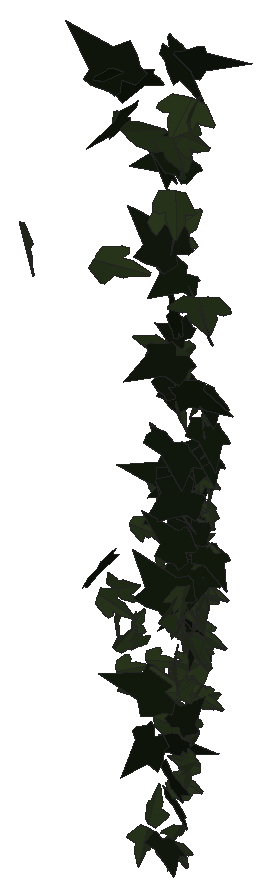
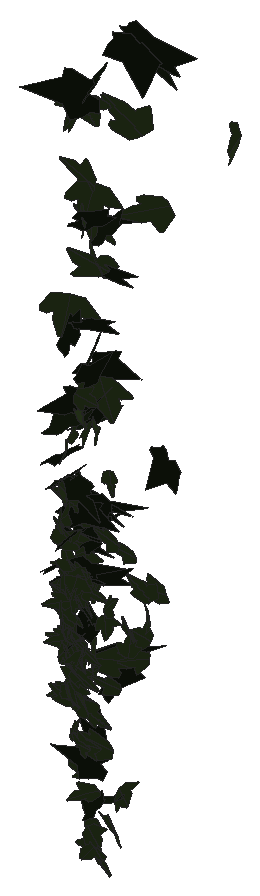
# SketchUp Ruby script. Lengths in inches.
U = 1.inch
M = Sketchup.active_model
def pt(a) = Geom::Point3d.new(a.map { |v| v * U })
def face(e, loops, mat)
  f = e.add_face(loops[0].map { |a| pt(a) })
  loops[1..].each { |l| e.add_face(l.map { |a| pt(a) }).erase! }
  f.material = f.back_material = mat if mat
  f
end
# faces: each face lists its corners as indices into pts; further lists are holes
def faces(e, pts, list, mat = nil) = list.each { |f| face(e, (f[0].is_a?(Array) ? f : [f]).map { |l| l.map { |i| pts[i] } }, mat) }
# xy, xz, yz: faces in a plane at the given z, y or x. An outline is a flat list of corners, or four numbers for a rectangle; further outlines are holes
def ring(l) = l.size == 4 ? [[l[0], l[1]], [l[2], l[1]], [l[2], l[3]], [l[0], l[3]]] : l.each_slice(2).to_a
def flat(e, list, mat, &to3) = list.each { |f| face(e, (f[0].is_a?(Array) ? f : [f]).map { |l| ring(l).map { |u, v| to3.(u, v) } }, mat) }
def xy(e, z, list, mat = nil) = flat(e, list, mat) { |x, y| [x, y, z] }
def xz(e, y, list, mat = nil) = flat(e, list, mat) { |x, z| [x, y, z] }
def yz(e, x, list, mat = nil) = flat(e, list, mat) { |y, z| [x, y, z] }
def lines(e, pts, list) = list.each { |a, b| e.add_line(pt(pts[a]), pt(pts[b])) }
# prism: a flat outline (further loops are holes) pulled along v
def prism(e, loops, v, mat = nil)
  f = face(e, loops, mat); d = Geom::Vector3d.new(v.map { |x| x * U })
  f.pushpull(f.normal.samedirection?(d) ? d.length : -d.length)
end
def box(e, o, s, mat = nil) = prism(e, [[o, [o[0] + s[0], o[1], o[2]], [o[0] + s[0], o[1] + s[1], o[2]], [o[0], o[1] + s[1], o[2]]]], [0, 0, s[2]], mat)
def at(x, y, z, deg = 0) = Geom::Transformation.translation(pt([x, y, z])) * Geom::Transformation.rotation(ORIGIN, Z_AXIS, deg.degrees)
def axes(o, x, y, z) = Geom::Transformation.new([*x, 0, *y, 0, *z, 0, *pt(o).to_a, 1])
def part(name) = M.definitions.add(name)
# library, detail: a bought-in or finely detailed component or shape, given as its bounding box
def library(name, o, s) = part(name).tap { |d| box(d.entities, o, s) }
def detail(e, o, s) = box(e.add_group.entities, o, s)
def put(e, d, t, mat = nil) = e.add_instance(d, t).tap { |i| i.material = mat if mat }
def group(e, t, mat = nil) = e.add_group.tap { |g| g.transformation = t; g.material = mat if mat }.entities
root = M.entities
M.materials.add("1026 AP 7946 SUNNY SIDE UP").color = [254, 231, 186]
M.materials.add("efeu1").color = [18, 25, 13]
M.materials.add("efeu2").color = [43, 57, 29]
c1 = part("ivyleaf_10")
p = [[0,0.5,-0.03],[-0.0625,2.02,-0.43],[-0.19,2.01,-0.46],[-0.54,1.05,-0.29],[-0.52,0.625,-0.18],[-0.83,0.76,-0.28],
  [-1.16,0.64,-0.33],[-1.15,0.33,-0.24],[-0.77,-0.39,0.02],[-0.3,-0.51,0.16],[0.04,-0.48,0.23],[-0.02,2.01,-0.4375],
  [-0.06,2.01,-0.43],[0.04,-0.49,0.23],[0.67,-0.49,0.14],[1.38,0.36,-0.2],[1.375,0.51,-0.24],[0.81,0.65,-0.19],
  [0.62,0.59,-0.15],[0.6,1.09,-0.28],[0.5,1.23,-0.31]]
faces(c1.entities,p,[[0,1,2,3,4,5,6,7,8,9,10],[11,12,0,13,14,15,16,17,18,19,20]],"efeu2")
c2 = part("ivyleaf_9")
p = [[1.54,2.16,1.25],[1.36,2.04,1.19],[-0.21,0.99,0.68],[-0.71,1.11,0.82],[-0.85,0.86,0.67],[-0.8,0.17,0.21],
  [-0.9,-0.01,0.1],[-0.67,-0.16,-0.02],[-0.08,-0.08,-0.05],[-0.03,-0.6,-0.4],[0.65,-0.88,-0.66],[0.83,-0.6,-0.49],
  [1.29,-0.42,-0.43],[1.8125,-0.07,-0.26],[1.21,0.44,0.15]]
faces(c2.entities,p,[[0,1,2,3,4,5,6,7,8,9,10,11,12,13,14]],"efeu1")
put(root,c1,axes([137.27,204.8,264.4375],[-0.21228,0.31455,-0.21083],[0.10791,-0.19506,-0.35356],[-0.58168,-0.15098,0.01135]),"1026 AP 7946 SUNNY SIDE UP")
put(root,c2,axes([138.43,205.78,256.27],[-0.14943,0.12354,-0.33542],[-0.27565,0.27548,0.16166],[0.47432,0.19902,-0.01172]),"1026 AP 7946 SUNNY SIDE UP")
put(root,c2,axes([138.74,206.35,267.0625],[-0.36936,0.26298,-0.15561],[0.1174,-0.13697,-0.3625],[-0.46341,-0.24431,0.0322]),"1026 AP 7946 SUNNY SIDE UP")
put(root,c1,axes([137.98,206.61,263.21],[-0.15297,-0.09398,-0.35608],[0.46781,0.17726,-0.13509],[0.31218,-0.31168,0.02796]),"1026 AP 7946 SUNNY SIDE UP")
put(root,c2,axes([138.58,207.46,251.5],[0.02682,-0.05486,-0.40252],[0.29455,-0.34272,0.05604],[-0.54547,-0.18777,0.01047]),"1026 AP 7946 SUNNY SIDE UP")
put(root,c2,axes([137.97,207.08,267.47],[-0.03931,0.10478,0.44908],[-0.49984,0.3029,-0.09214],[-0.49583,-0.31366,0.05728]),"1026 AP 7946 SUNNY SIDE UP")
put(root,c2,axes([138.1,207.17,267.54],[0.27569,0.29178,-0.14907],[-0.09098,-0.13573,-0.35095],[-0.50515,0.18368,-0.01815]),"1026 AP 7946 SUNNY SIDE UP")
put(root,c1,axes([138.1,207.79,248.85],[-0.05681,-0.25331,0.18976],[0.16619,-0.18576,-0.24103],[0.465,0.03545,0.10933]),"1026 AP 7946 SUNNY SIDE UP")
put(root,c1,axes([137.82,207.68,265.81],[-0.35908,-0.09139,0.2943],[0.45463,0.03082,0.24799],[-0.12835,0.36484,0.05505]),"1026 AP 7946 SUNNY SIDE UP")
put(root,c1,axes([137.11,207.7,254.25],[0.08937,0.02554,0.27361],[0.41558,0.03078,-0.06117],[-0.05589,0.26971,-0.01732]),"1026 AP 7946 SUNNY SIDE UP")
put(root,c2,axes([138.4,208,252.34],[-0.16035,-0.2823,-0.21493],[-0.10551,-0.19588,0.30806],[-0.54026,0.12204,0.00363]),"1026 AP 7946 SUNNY SIDE UP")
put(root,c1,axes([137.22,207.97,253.61],[-0.02174,0.04114,-0.24935],[0.1048,-0.23294,-0.04603],[-0.37193,-0.06804,0.0016]),"1026 AP 7946 SUNNY SIDE UP")
put(root,c1,axes([138.37,208.11,252.28],[-0.05152,0.0425,0.36196],[-0.31307,-0.29365,0.01575],[0.45962,-0.19525,0.0513]),"1026 AP 7946 SUNNY SIDE UP")
put(root,c2,axes([138.57,208.1875,258.29],[-0.07894,-0.35099,0.12447],[0.13846,-0.13162,-0.35122],[0.56808,-0.01669,0.1029]),"1026 AP 7946 SUNNY SIDE UP")
put(root,c2,axes([138.35,208.11,248.66],[-0.04833,-0.26842,0.06253],[0.14171,-0.06896,-0.261],[0.40942,-0.00781,0.09772]),"1026 AP 7946 SUNNY SIDE UP")
put(root,c1,axes([138.48,208.32,254.14],[0.01062,-0.05018,-0.36681],[-0.03601,-0.35517,0.04908],[-0.56381,0.02174,-0.01005]),"1026 AP 7946 SUNNY SIDE UP")
put(root,c2,axes([138.42,208.24,250.11],[0.07435,-0.07825,0.29064],[0.15266,-0.26589,-0.09415],[0.43502,0.10668,-0.01664]),"1026 AP 7946 SUNNY SIDE UP")
put(root,c1,axes([137.3125,207.95,253.1],[0.00959,-0.17395,0.17565],[-0.01251,0.17131,0.18031],[-0.38388,-0.00993,-0.00149]),"1026 AP 7946 SUNNY SIDE UP")
put(root,c1,axes([137.39,207.93,252.55],[0.02346,-0.01229,-0.25266],[0.24321,0.19122,0.00094],[0.29976,-0.15419,0.01902]),"1026 AP 7946 SUNNY SIDE UP")
put(root,c1,axes([137.14,208.11,254.33],[-0.25796,-0.01163,0.18737],[0.28374,0.02458,0.16938],[-0.04092,0.24375,-0.0067]),"1026 AP 7946 SUNNY SIDE UP")
put(root,c1,axes([138.48,208.48,248.2],[0.05216,-0.07558,0.20674],[0.08378,-0.19425,-0.08539],[0.32727,0.06177,-0.01109]),"1026 AP 7946 SUNNY SIDE UP")
put(root,c1,axes([138.76,208.4,266.45],[0.49856,0.13271,-0.10172],[-0.12513,-0.06662,-0.35318],[-0.22882,0.32557,-0.02851]),"1026 AP 7946 SUNNY SIDE UP")
put(root,c1,axes([137.41,208.43,252.96],[-0.12147,-0.17915,-0.06958],[-0.05431,-0.05748,0.20046],[-0.29553,0.08419,-0.00824]),"1026 AP 7946 SUNNY SIDE UP")
put(root,c1,axes([138.59,208.46,254.59],[-0.06434,-0.29395,0.07829],[0.11226,-0.08546,-0.29498],[0.4647,-0.02006,0.0821]),"1026 AP 7946 SUNNY SIDE UP")
put(root,c2,axes([138.61,208.45,255.63],[-0.2433,-0.28255,0.01311],[-0.00479,0.018,0.33177],[-0.44482,0.15435,-0.01075]),"1026 AP 7946 SUNNY SIDE UP")
put(root,c2,axes([138.47,208.375,254.44],[-0.47842,-0.18786,-0.0325],[-0.06268,0.00671,0.3674],[-0.29262,0.30571,-0.02557]),"1026 AP 7946 SUNNY SIDE UP")
put(root,c2,axes([138.2,208.64,260.1],[-0.00175,-0.01928,-0.36432],[-0.00079,-0.35353,0.0178],[-0.55672,0.00056,0.00112]),"1026 AP 7946 SUNNY SIDE UP")
put(root,c1,axes([137.35,208.43,253.39],[0.23057,-0.14791,-0.03381],[0.05167,-0.01234,0.21398],[-0.23227,-0.14957,0.01404]),"1026 AP 7946 SUNNY SIDE UP")
put(root,c2,axes([138.46,208.54,251.31],[-0.20919,0.18329,0.17464],[0.16876,-0.13014,0.2324],[0.35322,0.17073,-0.00761]),"1026 AP 7946 SUNNY SIDE UP")
put(root,c1,axes([138.45,208.38,252.74],[-0.08363,0.11263,0.31846],[-0.31206,0.23796,-0.12336],[-0.41143,-0.20338,0.02884]),"1026 AP 7946 SUNNY SIDE UP")
put(root,c1,axes([138.47,208.67,249.97],[-0.04252,-0.20025,0.02134],[0.07316,-0.02766,-0.20198],[0.30818,-0.02106,0.0509]),"1026 AP 7946 SUNNY SIDE UP")
put(root,c1,axes([137.17,208.6875,255.61],[0.00895,-0.03411,-0.21442],[0.30603,-0.07888,0.01836],[-0.12701,-0.19248,0.02912]),"1026 AP 7946 SUNNY SIDE UP")
put(root,c2,axes([138.48,208.8,256.82],[-0.58057,0.01593,-0.03948],[0.05748,-0.0392,-0.379],[-0.03116,-0.36914,0.03635]),"1026 AP 7946 SUNNY SIDE UP")
put(root,c1,axes([138.09,208.79,263.77],[0.52149,-0.09691,0.15922],[0.21566,-0.0807,-0.35453],[0.19025,0.35713,-0.03455]),"1026 AP 7946 SUNNY SIDE UP")
put(root,c1,axes([138.9,208.43,266.15],[-0.00558,0.03021,0.35349],[-0.21461,0.31475,-0.02818],[-0.49699,-0.13625,0.0082]),"1026 AP 7946 SUNNY SIDE UP")
put(root,c1,axes([138.43,208.61,249.625],[0.13704,0.21404,-0.06837],[0.02392,0.0667,0.23822],[0.35212,-0.08783,0.01043]),"1026 AP 7946 SUNNY SIDE UP")
put(root,c1,axes([138.38,208.68,253.75],[0.10194,-0.24117,-0.11016],[-0.03952,0.10254,-0.25666],[0.41206,0.0695,0.00263]),"1026 AP 7946 SUNNY SIDE UP")
put(root,c1,axes([138.36,208.78,252],[0.19521,-0.1543,-0.11315],[0.12625,-0.07491,0.2031],[-0.26885,-0.14721,0.01322]),"1026 AP 7946 SUNNY SIDE UP")
put(root,c1,axes([138.47,208.89,250.26],[-0.00801,0.05453,0.21713],[0.08596,-0.20343,0.05447],[0.33086,0.05417,-0.00889]),"1026 AP 7946 SUNNY SIDE UP")
put(root,c2,axes([138.16,208.6875,262.59],[-0.51837,-0.07034,-0.17757],[-0.27636,0.00448,0.34524],[-0.09474,0.3718,-0.0355]),"1026 AP 7946 SUNNY SIDE UP")
put(root,c2,axes([138.33,208.82,253.98],[-0.29779,0.13854,-0.10576],[0.11107,-0.07805,-0.24136],[-0.24815,-0.20119,0.01889]),"1026 AP 7946 SUNNY SIDE UP")
put(root,c1,axes([138.25,208.88,254.02],[0.09784,-0.00823,0.23936],[0.3392,-0.08777,-0.06322],[0.13651,0.22399,-0.01447]),"1026 AP 7946 SUNNY SIDE UP")
put(root,c2,axes([138.05,208.76,267.38],[0.36087,-0.28525,-0.21895],[-0.22656,0.1546,-0.37601],[0.50974,0.27066,-0.01211]),"1026 AP 7946 SUNNY SIDE UP")
put(root,c1,axes([138.47,208.84,251.4],[-0.35283,0.0622,0.10485],[0.16392,-0.00155,0.23858],[0.09016,0.24624,-0.02345]),"1026 AP 7946 SUNNY SIDE UP")
put(root,c1,axes([138.8,208.83,261.5],[-0.50005,-0.21165,-0.04949],[0.08921,-0.001,-0.39216],[0.32897,-0.32144,0.03111]),"1026 AP 7946 SUNNY SIDE UP")
put(root,c1,axes([137.88,209.04,263.09],[0.28789,-0.18585,0.2122],[0.21162,-0.15775,-0.26942],[0.38287,0.22694,-0.01064]),"1026 AP 7946 SUNNY SIDE UP")
put(root,c2,axes([137.87,209.04,249.07],[0.1098,-0.1935,0.14411],[0.06205,-0.13555,-0.21258],[0.3713,0.07987,-0.00709]),"1026 AP 7946 SUNNY SIDE UP")
put(root,c2,axes([137.99,208.9,259.16],[-0.1715,-0.24048,0.15713],[0.08622,0.14403,0.27274],[-0.44057,0.1218,-0.00779]),"1026 AP 7946 SUNNY SIDE UP")
put(root,c1,axes([138.01,209,248.43],[-0.08255,-0.19904,0.07055],[-0.01351,-0.06966,-0.21227],[0.33129,-0.05244,0.00892]),"1026 AP 7946 SUNNY SIDE UP")
put(root,c2,axes([138.11,208.96,256.86],[-0.20076,-0.07795,-0.23052],[-0.32185,-0.09077,0.15267],[-0.18639,0.2407,-0.01533]),"1026 AP 7946 SUNNY SIDE UP")
put(root,c1,axes([138.02,208.95,248.03],[-0.30631,0.03804,-0.0833],[0.11627,-0.04119,-0.20318],[-0.07945,-0.20694,0.02382]),"1026 AP 7946 SUNNY SIDE UP")
put(root,c1,axes([138.44,209.1,250.83],[-0.0274,0.05563,0.20616],[0.14152,-0.17861,0.05827],[0.29381,0.09122,-0.00884]),"1026 AP 7946 SUNNY SIDE UP")
put(root,c1,axes([138.47,208.98,253.125],[-0.38521,0.0857,-0.11891],[0.15772,-0.06281,-0.26661],[-0.1628,-0.26364,0.02307]),"1026 AP 7946 SUNNY SIDE UP")
put(root,c1,axes([138.47,209.02,253.18],[-0.29423,0.12034,-0.17806],[0.20782,-0.11408,-0.22899],[-0.25896,-0.22827,0.01854]),"1026 AP 7946 SUNNY SIDE UP")
put(root,c1,axes([138.08,209.05,256.44],[-0.03035,-0.0377,-0.25412],[0.34512,-0.11983,0.00048],[-0.18598,-0.21623,0.04236]),"1026 AP 7946 SUNNY SIDE UP")
put(root,c2,axes([138.17,208.84,259.2],[0.05089,0.00326,-0.32937],[0.24383,0.28089,0.02077],[0.43969,-0.15614,0.0266]),"1026 AP 7946 SUNNY SIDE UP")
put(root,c2,axes([138.48,208.85,255.64],[-0.52553,0.02145,-0.08664],[-0.12803,0.03973,0.34354],[0.04778,0.34237,-0.0324]),"1026 AP 7946 SUNNY SIDE UP")
put(root,c1,axes([137.92,208.92,247.87],[0.14845,-0.11689,-0.18783],[-0.20684,0.12614,-0.15331],[0.26943,0.16125,-0.01421]),"1026 AP 7946 SUNNY SIDE UP")
put(root,c1,axes([137.37,208.99,252.32],[0.09255,-0.02455,-0.20343],[0.31189,-0.00731,0.06185],[-0.02213,-0.20579,0.02085]),"1026 AP 7946 SUNNY SIDE UP")
put(root,c1,axes([137.41,208.93,248.5625],[0.3866,-0.19255,0.102],[-0.0914,0.08732,0.3206],[-0.32877,-0.25069,0.03081]),"1026 AP 7946 SUNNY SIDE UP")
put(root,c2,axes([138.38,209.29,260.89],[0.03261,-0.12433,0.39737],[0.08169,-0.38293,-0.13204],[0.63304,0.05582,-0.00343]),"1026 AP 7946 SUNNY SIDE UP")
put(root,c2,axes([138.14,209.12,253.43],[0.34432,-0.13217,0.017],[-0.00467,0.02834,0.26262],[-0.20953,-0.21782,0.02209]),"1026 AP 7946 SUNNY SIDE UP")
put(root,c1,axes([138.25,209.13,252.26],[-0.14705,-0.08734,-0.18617],[-0.21653,-0.11637,0.13104],[-0.22864,0.16638,-0.00436]),"1026 AP 7946 SUNNY SIDE UP")
put(root,c2,axes([137.9375,209.15,256.8],[-0.26336,0.02022,0.29029],[-0.4377,-0.06695,-0.16596],[0.07475,-0.32079,0.05097]),"1026 AP 7946 SUNNY SIDE UP")
put(root,c2,axes([138.39,209.18,254.79],[-0.27314,-0.2426,-0.05525],[0.07861,0.02826,-0.30624],[0.38221,-0.17918,0.0235]),"1026 AP 7946 SUNNY SIDE UP")
put(root,c1,axes([138.07,209,258.75],[-0.12102,0.27967,0.01811],[-0.02748,0.01176,-0.29842],[-0.43962,-0.07773,0.01367]),"1026 AP 7946 SUNNY SIDE UP")
put(root,c1,axes([138.39,209.07,250.09],[0.02983,-0.01261,-0.20835],[-0.31353,0.03459,-0.0213],[0.05608,0.20009,-0.00824]),"1026 AP 7946 SUNNY SIDE UP")
put(root,c1,axes([137.68,209.08,259.9],[-0.56075,-0.06376,0.13403],[-0.19072,-0.05944,-0.37182],[0.12556,-0.37506,0.03383]),"1026 AP 7946 SUNNY SIDE UP")
put(root,c1,axes([138.44,209.05,251.87],[-0.19637,-0.05084,-0.21241],[0.32776,0.01461,-0.13388],[0.06145,-0.24036,0.03531]),"1026 AP 7946 SUNNY SIDE UP")
put(root,c2,axes([138.03,209.2,255.81],[0.26522,-0.22788,0.09308],[-0.06293,0.08419,0.29203],[-0.38104,-0.17251,0.01655]),"1026 AP 7946 SUNNY SIDE UP")
put(root,c1,axes([137.33,209.26,254.44],[0.00113,0.02169,0.22004],[0.11205,-0.20137,0.01965],[0.31823,0.07083,-0.0077]),"1026 AP 7946 SUNNY SIDE UP")
put(root,c1,axes([138.37,209.2,253.33],[-0.00667,-0.19743,-0.10454],[-0.00697,-0.10028,0.20284],[-0.34817,0.00579,-0.00206]),"1026 AP 7946 SUNNY SIDE UP")
put(root,c1,axes([138.09,209.13,254.63],[-0.10759,0.00135,0.20859],[-0.30217,-0.06775,-0.06684],[0.10027,-0.2027,0.02241]),"1026 AP 7946 SUNNY SIDE UP")
put(root,c1,axes([137.53,209.16,250.82],[0.00838,-0.03053,-0.31371],[0.45089,-0.10543,0.01545],[-0.16737,-0.28555,0.02592]),"1026 AP 7946 SUNNY SIDE UP")
put(root,c2,axes([138,209.02,260.53],[-0.0697,-0.16956,0.25995],[0.07994,0.24826,0.18182],[-0.47256,0.067,-0.00758]),"1026 AP 7946 SUNNY SIDE UP")
put(root,c1,axes([137.76,208.97,262.82],[0.37546,0.07194,-0.27499],[0.35066,0.15922,0.25027],[0.25797,-0.32115,0.06004]),"1026 AP 7946 SUNNY SIDE UP")
put(root,c1,axes([138.38,209.17,252.47],[0.28959,-0.04065,-0.18182],[-0.28037,0.00158,-0.1923],[0.04792,0.25492,-0.02628]),"1026 AP 7946 SUNNY SIDE UP")
put(root,c1,axes([138.38,209.22,253.95],[0.28876,-0.09256,0.11789],[0.14727,-0.06875,-0.21156],[0.17936,0.20546,-0.0161]),"1026 AP 7946 SUNNY SIDE UP")
put(root,c1,axes([138.04,209.15,255.45],[-0.14781,-0.20461,-0.00666],[0.01645,0.00103,-0.23177],[0.32141,-0.09415,0.0088]),"1026 AP 7946 SUNNY SIDE UP")
put(root,c1,axes([138.53,209.18,252.02],[0.09617,-0.20196,0.00355],[-0.00711,-0.00617,-0.21734],[0.31757,0.06102,-0.00594]),"1026 AP 7946 SUNNY SIDE UP")
put(root,c1,axes([138.14,209.31,254.52],[-0.03365,-0.24586,0.17407],[0.14595,-0.16783,-0.23848],[0.44711,0.03628,0.09095]),"1026 AP 7946 SUNNY SIDE UP")
put(root,c1,axes([138.4375,209.15,251.99],[-0.31393,0.00268,0.13484],[-0.20426,-0.03339,-0.20366],[0.02529,-0.23637,0.02889]),"1026 AP 7946 SUNNY SIDE UP")
put(root,c1,axes([137.91,209.22,265.09],[-0.10024,0.05344,0.33373],[0.50792,-0.04715,0.07329],[0.08976,0.32648,-0.04204]),"1026 AP 7946 SUNNY SIDE UP")
put(root,c1,axes([138.51,209.13,251.66],[-0.20743,-0.06641,0.15099],[0.19357,0.08114,0.15211],[-0.16377,0.18003,-0.01145]),"1026 AP 7946 SUNNY SIDE UP")
put(root,c1,axes([137.4,209.11,257.72],[-0.23451,0.09458,0.10549],[-0.15171,0.03711,-0.18081],[-0.15733,-0.17675,0.01711]),"1026 AP 7946 SUNNY SIDE UP")
put(root,c1,axes([138.51,209.31,253.09],[-0.02854,-0.22591,0.12697],[0.12494,-0.12366,-0.2199],[0.38589,0.02333,0.08059]),"1026 AP 7946 SUNNY SIDE UP")
put(root,c1,axes([138.59,209.22,253.79],[0.05508,-0.26684,0.00737],[0.07168,-0.00264,-0.27339],[0.41363,0.03599,0.0464]),"1026 AP 7946 SUNNY SIDE UP")
put(root,c1,axes([137.63,209.33,258.85],[-0.06233,0.0565,-0.20028],[0.0231,-0.1971,-0.06314],[-0.31799,-0.02539,0.03467]),"1026 AP 7946 SUNNY SIDE UP")
put(root,c1,axes([138.32,209.23,253.28],[-0.12799,-0.00103,-0.25664],[0.37376,-0.07876,-0.08013],[-0.11723,-0.24996,0.0247]),"1026 AP 7946 SUNNY SIDE UP")
put(root,c2,axes([137.7,209.14,250.34],[0.25443,0.09029,-0.20688],[0.24878,0.12656,0.1902],[0.24184,-0.22517,0.022]),"1026 AP 7946 SUNNY SIDE UP")
put(root,c2,axes([138.16,209.28,255.18],[-0.14871,0.02877,0.25893],[-0.39737,-0.01848,-0.09595],[0.01145,-0.26775,0.03285]),"1026 AP 7946 SUNNY SIDE UP")
put(root,c2,axes([137.875,209.36,260.1],[0.01651,0.04137,0.27628],[-0.31028,-0.18272,0.03596],[0.29236,-0.19626,0.02257]),"1026 AP 7946 SUNNY SIDE UP")
put(root,c2,axes([138.22,208.97,267.11],[0.15505,0.19314,-0.30545],[0.14599,0.28406,0.22328],[0.53841,-0.13265,0.02742]),"1026 AP 7946 SUNNY SIDE UP")
put(root,c2,axes([138.24,209.3,253.04],[-0.2258,0.02543,-0.20214],[0.29315,-0.06431,-0.14942],[-0.10483,-0.23461,0.01755]),"1026 AP 7946 SUNNY SIDE UP")
put(root,c2,axes([138.13,209.35,256.77],[0.0173,0.01721,-0.30082],[-0.14744,-0.27669,-0.02205],[-0.43584,0.09429,-0.00448]),"1026 AP 7946 SUNNY SIDE UP")
put(root,c1,axes([138.21,209.17,253.1],[-0.07953,0.04606,0.23509],[-0.36306,0.0178,-0.05638],[-0.0435,-0.2328,0.04077]),"1026 AP 7946 SUNNY SIDE UP")
put(root,c1,axes([138.35,209.26,252.87],[0.27702,-0.00684,0.14989],[0.22711,-0.02185,-0.1813],[0.03015,0.22747,-0.01156]),"1026 AP 7946 SUNNY SIDE UP")
put(root,c1,axes([137.92,209.09,249.52],[0.07426,0.10325,0.20814],[0.16338,0.17294,-0.1154],[-0.31624,0.1136,-0.01074]),"1026 AP 7946 SUNNY SIDE UP")
put(root,c1,axes([138.04,209.16,255.79],[0.05603,-0.02812,-0.23275],[0.35076,0.04924,0.03024],[0.07032,-0.2232,0.03461]),"1026 AP 7946 SUNNY SIDE UP")
put(root,c1,axes([138.34,209.2,253.28],[-0.20914,-0.03793,-0.23237],[0.35791,0.00099,-0.13858],[0.03168,-0.26167,0.0316]),"1026 AP 7946 SUNNY SIDE UP")
put(root,c1,axes([138.22,209.32,253.04],[-0.06811,-0.20709,0.07854],[-0.01812,-0.07667,-0.21837],[0.34717,-0.04463,0.00401]),"1026 AP 7946 SUNNY SIDE UP")
put(root,c2,axes([138.38,209.47,257.47],[-0.08463,-0.24425,0.13328],[-0.0324,-0.1293,-0.25833],[0.43443,-0.05723,0.0067]),"1026 AP 7946 SUNNY SIDE UP")
put(root,c1,axes([138.22,209.18,250.63],[0.1471,-0.0091,0.18546],[-0.26449,0.06866,0.094],[-0.1021,-0.19096,0.0237]),"1026 AP 7946 SUNNY SIDE UP")
put(root,c2,axes([137.84,209.44,261.6],[-0.35307,-0.14727,0.09312],[-0.09906,-0.0697,-0.27607],[0.25375,-0.23213,0.02179]),"1026 AP 7946 SUNNY SIDE UP")
put(root,c1,axes([138.08,209.16,254.75],[0.0787,0.06554,0.27322],[0.33914,0.15539,-0.0807],[-0.26272,0.22022,-0.02233]),"1026 AP 7946 SUNNY SIDE UP")
put(root,c1,axes([137.78,209.24,264.86],[-0.46736,-0.20512,-0.06827],[0.11081,0.01211,-0.37072],[0.31972,-0.30403,0.0287]),"1026 AP 7946 SUNNY SIDE UP")
put(root,c1,axes([137.39,209.27,254.12],[-0.12489,-0.19033,-0.01484],[0.02013,0.00908,-0.21224],[0.29933,-0.08002,0.00808]),"1026 AP 7946 SUNNY SIDE UP")
put(root,c1,axes([138.16,209.29,253.14],[0.27677,-0.11958,-0.10719],[0.15167,-0.0413,0.21819],[-0.19689,-0.1999,0.0174]),"1026 AP 7946 SUNNY SIDE UP")
put(root,c2,axes([137.14,209.53,264.15],[0.01876,-0.23778,0.25573],[0.06603,-0.24687,-0.24581],[0.53801,0.03859,0.02125]),"1026 AP 7946 SUNNY SIDE UP")
put(root,c2,axes([138.5625,209.36,255.22],[0.04581,-0.26859,-0.05813],[0.04512,0.05789,-0.27576],[0.4287,0.02261,0.03523]),"1026 AP 7946 SUNNY SIDE UP")
put(root,c1,axes([137.99,209.21,250.71],[0.20432,-0.01213,0.21302],[-0.31206,0.06288,0.1326],[-0.09363,-0.23604,0.0229]),"1026 AP 7946 SUNNY SIDE UP")
put(root,c1,axes([138.4,209.37,254.68],[0.18094,-0.14996,0.07521],[0.05311,-0.06696,-0.19466],[0.25742,0.11922,-0.0127]),"1026 AP 7946 SUNNY SIDE UP")
put(root,c1,axes([138.48,209.31,253.04],[0.22045,-0.20473,-0.04466],[-0.0452,0.03144,-0.25537],[0.32555,0.143,-0.00521]),"1026 AP 7946 SUNNY SIDE UP")
put(root,c1,axes([137.09,209.39,256.28],[-0.00374,-0.01713,-0.2394],[0.29309,-0.13942,0.00781],[-0.21959,-0.1858,0.0145]),"1026 AP 7946 SUNNY SIDE UP")
put(root,c2,axes([138.33,209.51,255.91],[0.08252,-0.18739,-0.16739],[0.08101,-0.15311,0.19947],[-0.38037,-0.07326,0.00617]),"1026 AP 7946 SUNNY SIDE UP")
put(root,c2,axes([138.2,209.41,253.3125],[0.11182,-0.24839,0.0081],[-0.00549,-0.01065,-0.26615],[0.3908,0.07092,-0.00606]),"1026 AP 7946 SUNNY SIDE UP")
put(root,c1,axes([138.55,209.3,254.1],[0.04273,-0.24952,-0.06149],[0.04189,0.06103,-0.25608],[0.40072,0.02023,0.03333]),"1026 AP 7946 SUNNY SIDE UP")
put(root,c1,axes([137.96,209.28,251.6875],[0.13643,-0.22824,0.07826],[-0.02997,0.07536,0.25183],[-0.3777,-0.08842,0.00829]),"1026 AP 7946 SUNNY SIDE UP")
put(root,c1,axes([138.17,209.47,258.65],[-0.10136,0.14026,0.23838],[0.17356,-0.20265,0.15759],[0.38728,0.12753,-0.00823]),"1026 AP 7946 SUNNY SIDE UP")
put(root,c2,axes([138.1875,209.59,258.9375],[-0.04021,-0.33195,0.15851],[0.17672,-0.1557,-0.32378],[0.5488,0.02582,0.11587]),"1026 AP 7946 SUNNY SIDE UP")
put(root,c1,axes([138.42,209.39,254.9],[-0.01383,-0.21192,0.02336],[0.05872,-0.02506,-0.2151],[0.33015,-0.00442,0.03923]),"1026 AP 7946 SUNNY SIDE UP")
put(root,c1,axes([138.2,209.34,254.86],[-0.30711,-0.07713,-0.03686],[0.06278,-0.0053,-0.21544],[0.11771,-0.19841,0.01874]),"1026 AP 7946 SUNNY SIDE UP")
put(root,c2,axes([138.46,209.48,258.08],[-0.02813,-0.29556,-0.01932],[0.00748,0.01682,-0.30492],[0.46545,-0.01814,0.00373]),"1026 AP 7946 SUNNY SIDE UP")
put(root,c1,axes([138.26,209.36,255.22],[0.31529,0.11018,0.06576],[0.10314,0.01132,-0.23465],[-0.17104,0.20994,-0.02028]),"1026 AP 7946 SUNNY SIDE UP")
put(root,c1,axes([138.2,209.42,256.91],[-0.01874,0.03169,0.27053],[0.4089,-0.04568,0.01758],[0.07451,0.25869,-0.02846]),"1026 AP 7946 SUNNY SIDE UP")
put(root,c1,axes([138.36,209.33,254.33],[0.23779,-0.01871,-0.14161],[0.21759,0.00848,0.15582],[-0.01275,-0.20412,0.01825]),"1026 AP 7946 SUNNY SIDE UP")
put(root,c1,axes([137.85,209.28,251.69],[0.05315,-0.05218,-0.27628],[-0.34211,0.15781,-0.05903],[0.25908,0.21909,-0.02126]),"1026 AP 7946 SUNNY SIDE UP")
put(root,c1,axes([138.04,209.36,253.11],[0.04148,0.2593,-0.01137],[0.00026,-0.01259,-0.26858],[-0.40821,0.02634,-0.00132]),"1026 AP 7946 SUNNY SIDE UP")
put(root,c1,axes([138.375,209.33,254.3],[-0.17157,-0.04504,-0.20686],[0.31348,0.03202,-0.11897],[0.07859,-0.22605,0.02296]),"1026 AP 7946 SUNNY SIDE UP")
put(root,c1,axes([138.39,209.22,253.63],[0.03298,-0.0578,-0.23101],[-0.02694,0.22382,-0.05987],[0.36262,0.02188,0.01656]),"1026 AP 7946 SUNNY SIDE UP")
put(root,c1,axes([137.75,209.6,264.23],[-0.00569,0.01709,-0.31126],[0.06529,-0.29937,-0.01971],[-0.4715,-0.04166,0.00103]),"1026 AP 7946 SUNNY SIDE UP")
put(root,c1,axes([137.84,209.53,259.13],[-0.05649,-0.08596,-0.18651],[0.09264,-0.17985,0.07508],[-0.30048,-0.03929,0.05821]),"1026 AP 7946 SUNNY SIDE UP")
put(root,c2,axes([138.39,209.53,257.41],[-0.0159,-0.23965,0.04806],[0.06814,-0.04905,-0.24311],[0.37823,-0.00124,0.04582]),"1026 AP 7946 SUNNY SIDE UP")
put(root,c1,axes([138.27,209.43,255.3],[-0.08503,-0.21874,0.00067],[0.00613,0.00099,0.23211],[-0.34391,0.0541,0.00397]),"1026 AP 7946 SUNNY SIDE UP")
put(root,c2,axes([137.77,209.63,264.31],[-0.34391,-0.11219,0.25634],[-0.32041,-0.14625,-0.25266],[0.28692,-0.29779,0.0251]),"1026 AP 7946 SUNNY SIDE UP")
put(root,c1,axes([138.41,209.48,256.15],[0.21466,-0.03943,0.15551],[0.21485,-0.06723,-0.14557],[0.11913,0.19228,-0.01769]),"1026 AP 7946 SUNNY SIDE UP")
put(root,c1,axes([138.43,209.57,256.36],[0.03866,-0.02829,0.21701],[0.191,-0.17233,-0.03943],[0.27454,0.12387,-0.00312]),"1026 AP 7946 SUNNY SIDE UP")
put(root,c1,axes([138.34,209.5,258.23],[-0.05594,0.1645,-0.13667],[0.03642,-0.13164,-0.17411],[-0.33122,-0.04225,0.00394]),"1026 AP 7946 SUNNY SIDE UP")
put(root,c2,axes([138.12,209.4,257.45],[-0.16635,0.26133,-0.10776],[0.04669,-0.10235,-0.29085],[-0.44101,-0.10941,0.00986]),"1026 AP 7946 SUNNY SIDE UP")
put(root,c1,axes([138.27,209.59,256.57],[-0.01944,0.03958,0.22891],[0.11961,-0.20855,0.04145],[0.33376,0.07704,-0.00152]),"1026 AP 7946 SUNNY SIDE UP")
put(root,c1,axes([138.36,209.57,257.28],[0.08056,-0.17401,0.15699],[0.06514,-0.14769,-0.18773],[0.35887,0.06587,-0.00117]),"1026 AP 7946 SUNNY SIDE UP")
put(root,c1,axes([138.4375,209.5,255.87],[-0.20158,-0.07622,-0.15653],[-0.21995,-0.05987,0.15262],[-0.1508,0.18922,-0.01336]),"1026 AP 7946 SUNNY SIDE UP")
put(root,c1,axes([138.22,209.46,253.93],[-0.09975,0.02906,0.20414],[0.31358,-0.00808,0.067],[0.02615,0.20775,-0.02471]),"1026 AP 7946 SUNNY SIDE UP")
put(root,c1,axes([137.85,209.57,259.78],[-0.03777,-0.1374,0.18172],[-0.04157,-0.17521,-0.1447],[0.35009,-0.03563,0.00243]),"1026 AP 7946 SUNNY SIDE UP")
